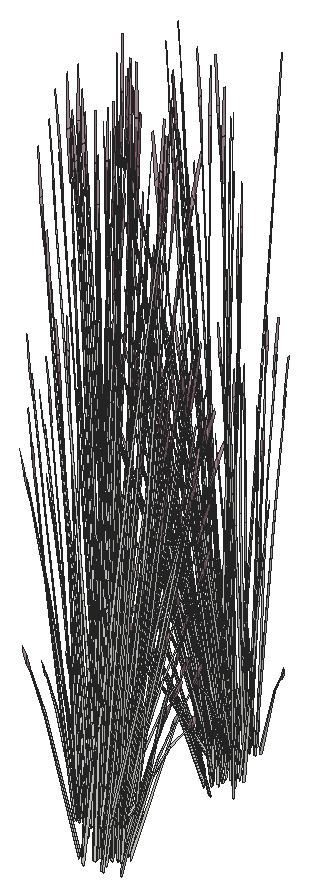
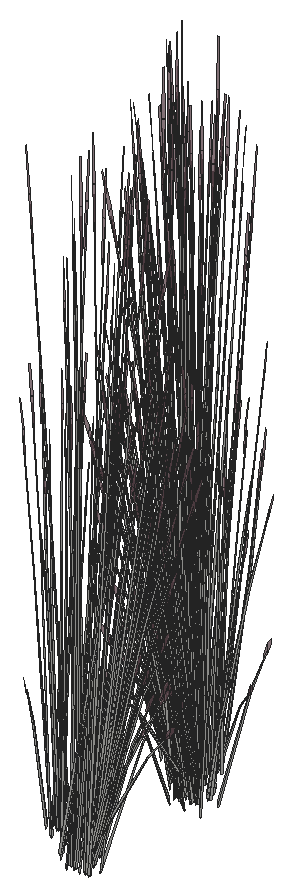
# SketchUp Ruby script. Lengths in inches.
U = 1.inch
M = Sketchup.active_model
def pt(a) = Geom::Point3d.new(a.map { |v| v * U })
def face(e, loops, mat)
  f = e.add_face(loops[0].map { |a| pt(a) })
  loops[1..].each { |l| e.add_face(l.map { |a| pt(a) }).erase! }
  f.material = f.back_material = mat if mat
  f
end
# faces: each face lists its corners as indices into pts; further lists are holes
def faces(e, pts, list, mat = nil) = list.each { |f| face(e, (f[0].is_a?(Array) ? f : [f]).map { |l| l.map { |i| pts[i] } }, mat) }
# xy, xz, yz: faces in a plane at the given z, y or x. An outline is a flat list of corners, or four numbers for a rectangle; further outlines are holes
def ring(l) = l.size == 4 ? [[l[0], l[1]], [l[2], l[1]], [l[2], l[3]], [l[0], l[3]]] : l.each_slice(2).to_a
def flat(e, list, mat, &to3) = list.each { |f| face(e, (f[0].is_a?(Array) ? f : [f]).map { |l| ring(l).map { |u, v| to3.(u, v) } }, mat) }
def xy(e, z, list, mat = nil) = flat(e, list, mat) { |x, y| [x, y, z] }
def xz(e, y, list, mat = nil) = flat(e, list, mat) { |x, z| [x, y, z] }
def yz(e, x, list, mat = nil) = flat(e, list, mat) { |y, z| [x, y, z] }
def lines(e, pts, list) = list.each { |a, b| e.add_line(pt(pts[a]), pt(pts[b])) }
# prism: a flat outline (further loops are holes) pulled along v
def prism(e, loops, v, mat = nil)
  f = face(e, loops, mat); d = Geom::Vector3d.new(v.map { |x| x * U })
  f.pushpull(f.normal.samedirection?(d) ? d.length : -d.length)
end
def box(e, o, s, mat = nil) = prism(e, [[o, [o[0] + s[0], o[1], o[2]], [o[0] + s[0], o[1] + s[1], o[2]], [o[0], o[1] + s[1], o[2]]]], [0, 0, s[2]], mat)
def at(x, y, z, deg = 0) = Geom::Transformation.translation(pt([x, y, z])) * Geom::Transformation.rotation(ORIGIN, Z_AXIS, deg.degrees)
def axes(o, x, y, z) = Geom::Transformation.new([*x, 0, *y, 0, *z, 0, *pt(o).to_a, 1])
def part(name) = M.definitions.add(name)
# library, detail: a bought-in or finely detailed component or shape, given as its bounding box
def library(name, o, s) = part(name).tap { |d| box(d.entities, o, s) }
def detail(e, o, s) = box(e.add_group.entities, o, s)
def put(e, d, t, mat = nil) = e.add_instance(d, t).tap { |i| i.material = mat if mat }
def group(e, t, mat = nil) = e.add_group.tap { |g| g.transformation = t; g.material = mat if mat }.entities
root = M.entities
M.materials.add("LightPink_Translucent").color = [144, 107, 117]
M.materials["LightPink_Translucent"].alpha = 0.75
c1 = part("blade")
p = [[2.15,0.21,22],[0,0.17,0],[0.09,0.45,0],[2.18,0.31,22],[2.29,0.31,22],[0.38,0.45,0],
  [2.48,0.24,33],[2.49,0.24,33],[2.48,0.22,33]]
faces(c1.entities,p,[[0,1,2,3],[4,5,2,3],[6,3,4,7],[8,0,3,6]])
c2 = part("seeds")
p = [[0.3,-0.1,1.38],[-0.01,-0.03,1.59],[-0.01,-0.03,0.03],[0.14,-0.07,-0.07],[0.29,-0.03,3],[0.15,0.01,3.11]]
faces(c2.entities,p,[[0,1,2,3],[1,0,4,5]],"LightPink_Translucent")
c3 = part("blade with seeds")
put(c3.entities,c1,at(0,0,0))
put(c3.entities,c2,axes([2.4,0.25,30.99],[1.5799,-0.05474,1.17369],[-0.12525,1.92788,0.29478],[-0.07173,-0.02425,1.56792]))
put(root,c3,axes([331.12,469.75,1400.36],[-0.29264,0.42323,0.45755],[-0.34767,-0.3736,0.17955],[0.07055,-0.04224,1.58856]))
put(root,c3,axes([331.44,470.5,1400.3],[-0.32829,-0.4014,-0.06131],[0.32849,-0.40164,0],[-0.01146,-0.01402,1.75571]))
put(root,c3,axes([330.61,469.05,1400.47],[-0.10196,0.46348,0.17642],[-0.3731,-0.13116,0.35086],[0.06445,-0.00226,1.60407]))
put(root,c3,axes([332.47,470.56,1403.05],[-0.29332,-0.1301,0.35414],[0.08555,-0.37955,-0.4572],[0.11809,-0.0348,0.87481]))
put(root,c3,axes([329.4,469.86,1402.73],[0.09971,-0.42522,0.48003],[0.32782,0.1454,0.3958],[-0.12892,0.02555,0.9933]))
put(root,c3,axes([330.46,469.42,1399.59],[-0.3474,0.18671,1.28929],[-0.11057,-0.53572,0.50096],[0.21332,0.00891,1.46642]))
put(root,c3,axes([331.39,469.56,1400.62],[0.06809,-0.4162,0.1448],[0.33266,0.07225,-0.41347],[0.06054,0.04274,1.26744]))
put(root,c3,axes([329.37,469.75,1402.73],[-0.12963,-0.31798,0.0643],[0.23638,-0.15564,0.50621],[-0.1042,0.03071,0.77189]))
put(root,c3,axes([330.82,470.55,1400.36],[0.44609,0.09826,0.45755],[-0.09078,0.55493,0.17955],[-0.06519,-0.05359,1.58856]))
put(root,c3,axes([333.17,470.15,1399.49],[-0.01845,-0.0708,1.76342],[0.12793,-0.41416,-0.26939],[0.12905,-0.00596,0.30037]))
put(root,c3,axes([329.36,470.08,1399.49],[0.00895,0.0735,1.76342],[-0.18044,0.38382,-0.26939],[-0.12817,-0.01935,0.30037]))
put(root,c3,axes([331.25,469.67,1400.72],[-0.21202,-0.39143,0.44739],[0.32115,-0.27564,-0.21531],[0.06861,0.04843,1.43643]))
put(root,c3,axes([330.15,471.46,1400.03],[-0.08291,-0.40636,-0.30978],[0.32928,-0.11539,0.30978],[-0.06638,-0.04686,1.38974]))
put(root,c3,axes([330.58,471.44,1400.47],[0.37926,-0.12378,0.17642],[0.09365,0.46065,0.35086],[-0.03382,-0.06712,1.60407]))
put(root,c3,axes([331.36,469.7,1400.67],[0.35635,-0.30962,-0.29095],[0.23697,0.43749,-0.50002],[0.08792,0.04443,1.59708]))
put(root,c3,axes([332.78,470.52,1402.53],[0.29332,0.1301,-0.35414],[-0.08555,0.37955,0.4572],[0.11809,-0.0348,0.87481]))
put(root,c3,axes([330.0625,471.64,1400.02],[-0.33032,-0.23318,-0.49651],[0.19744,-0.41812,0],[-0.07523,-0.05311,1.57504]))
put(root,c3,axes([332.26,468.88,1400.02],[0.33032,0.23318,-0.49651],[-0.19744,0.41812,0],[0.07523,0.05311,1.57504]))
put(root,c3,axes([329.33,469.91,1402.53],[-0.29332,-0.1301,-0.35414],[0.08555,-0.37955,0.4572],[-0.11809,0.0348,0.87481]))
put(root,c3,axes([331.63,470.21,1400.21],[0.39487,0,0],[0,0.48281,0],[0,0,1.78407]))
put(root,c3,axes([330.96,470.82,1400.67],[-0.35635,0.30962,-0.29095],[-0.23697,-0.43749,-0.50002],[-0.08792,-0.04443,1.59708]))
put(root,c3,axes([331.74,469.08,1400.47],[-0.37926,0.12378,0.17642],[-0.09365,-0.46065,0.35086],[0.03382,0.06712,1.60407]))
put(root,c3,axes([331.98,470.05,1401.875],[-0.14639,0.01056,1.71376],[0.09712,-0.45778,0.13857],[0.20862,0.02831,0.73262]))
put(root,c3,axes([332.17,469.05,1400.03],[0.08291,0.40636,-0.30978],[-0.32928,0.11539,0.30978],[0.06638,0.04686,1.38974]))
put(root,c3,axes([332.73,470.68,1402.73],[0.12963,0.31798,0.0643],[-0.23638,0.15564,0.50621],[0.1042,-0.03071,0.77189]))
put(root,c3,axes([331.5,469.96,1400.38],[-0.44609,-0.09826,0.49198],[0.09078,-0.55493,0.19306],[0.06519,0.05359,1.70813]))
put(root,c3,axes([332.71,470.5625,1402.73],[-0.09971,0.42522,0.48003],[-0.32782,-0.1454,0.3958],[0.12892,-0.02555,0.9933]))
put(root,c3,axes([331.15,471.33,1400.2],[-0.11516,-0.40207,0],[0.32884,-0.1408,0],[0,0,1.54371]))
put(root,c3,axes([330.93,470.95,1400.62],[-0.06809,0.4162,0.1448],[-0.33266,-0.07225,-0.41347],[-0.06054,-0.04274,1.26744]))
put(root,c3,axes([329.64,469.87,1403.05],[0.29332,0.1301,0.35414],[-0.08555,0.37955,-0.4572],[-0.11809,0.0348,0.87481]))
put(root,c3,axes([331.58,471.27,1400.18],[0.37054,-0.15823,-0.19198],[0.1302,0.45581,0.00008],[0.0409,-0.01749,1.73897]))
put(root,c3,axes([331.71,471.47,1400.47],[0.10196,-0.46348,0.17642],[0.3731,0.13116,0.35086],[-0.06445,0.00226,1.60407]))
put(root,c3,axes([331.62,470.41,1400.21],[0.24637,0.30123,0],[-0.24637,0.30123,0],[0,0,1.69266]))
put(root,c3,axes([330.22,469.85,1401.34],[0.10032,-0.06746,1.77064],[0.0346,0.47103,0.13857],[-0.2173,0.0625,0.63284]))
put(root,c3,axes([332.29,470.28,1400.47],[-0.2773,-0.3397,0.17642],[0.27945,-0.32949,0.35086],[-0.03063,0.06937,1.60407]))
put(root,c3,axes([331.78,469.77,1400.06],[0.36714,0.07646,-0.62353],[-0.07747,0.47163,-0.16365],[0.10956,0.05715,1.37633]))
put(root,c3,axes([333.4,470.59,1400.77],[-0.21807,0.07699,1.1486],[0.10265,-0.31819,0.84392],[0.11568,0.02177,0.25299]))
put(root,c3,axes([331.07,471.51,1400.2],[-0.35581,-0.20937,0],[0.17124,-0.43505,0],[0,0,1.62707]))
put(root,c3,axes([331.36,470.96,1400.46],[-0.34464,-0.37536,-0.25192],[0.29,-0.42149,0.5513],[-0.0928,0.04391,1.68216]))
put(root,c3,axes([330.45,471.68,1400.48],[0.33032,0.23318,0.49651],[-0.19744,0.41812,0],[-0.07523,-0.05311,1.57504]))
put(root,c3,axes([331.62,470.0625,1400.72],[0.17124,-0.42022,0.44739],[0.35581,0.20224,-0.21531],[0,0.09687,1.43643]))
put(root,c3,axes([333.3,471.94,1402.71],[-0.03191,-0.04083,1.77383],[0.06981,-0.43764,-0.16761],[0.12571,-0.02796,0.31391]))
put(root,c3,axes([329.14,470.16,1402.72],[-0.05763,0.06055,1.74944],[0.0049,0.44239,-0.27667],[-0.13211,0.05753,0.14031]))
put(root,c3,axes([331.55,470.3,1400.29],[0,0.53934,-0.05637],[-0.44133,0,0],[0,0.01695,1.79368]))
put(root,c3,axes([329.53,470.11,1402.68],[-0.09562,0.42421,-0.51099],[-0.32782,-0.1454,-0.3958],[-0.13199,0.0389,0.97773]))
put(root,c3,axes([329.51,469.74,1403.03],[0.17758,0.42229,-0.1216],[-0.31518,0.20752,-0.67495],[-0.13282,0.05572,1.02557]))
put(root,c3,axes([331.58,469.92,1400.21],[0.21202,0.39143,-0.44739],[-0.32115,0.27564,0.21531],[0.06861,0.04843,1.43643]))
put(root,c3,axes([333.02,471.57,1401.93],[-0.06755,-0.39203,-0.03492],[0.31928,-0.09013,-0.15832],[0.06667,0.02485,0.52218]))
put(root,c3,axes([330.26,471.92,1400.375],[-0.22066,0.46731,0],[-0.36918,-0.26061,-0.51607],[-0.08408,-0.05936,1.63711]))
put(root,c3,axes([332.19,471.5625,1403.03],[0.0189,-0.47427,-0.1216],[0.35781,0.01296,-0.67495],[0.13781,0.03295,1.02557]))
put(root,c3,axes([332.52,470.3,1400.48],[0,-0.46636,0.49651],[0.39487,0,0],[0,0.10622,1.57504]))
put(root,c3,axes([331.53,470.64,1400.72],[0.38326,-0.02879,0.44739],[0.03466,0.47788,-0.21531],[-0.06861,0.04843,1.43643]))
put(root,c3,axes([331.77,470.16,1400.62],[0.32884,-0.136,0.1448],[0.11516,0.38837,-0.41347],[0,0.08547,1.26744]))
put(root,c3,axes([332.14,471.38,1403.05],[-0.20082,-0.29199,0.35414],[0.2293,-0.2764,-0.4572],[0.1165,0.04206,0.87481]))
put(root,c3,axes([331.1875,470.875,1400.21],[-0.38326,0.02879,-0.44739],[-0.03466,-0.47788,0.21531],[-0.06861,0.04843,1.43643]))
put(root,c3,axes([332.99,471.1,1400.59],[-0.085,-0.1147,1.43002],[0.1106,-0.37943,-0.30754],[0.17198,0.0514,0.61141]))
put(root,c3,axes([331.47,471.52,1400.2],[0.35581,0.20937,0],[-0.17124,0.43505,0],[0,0,1.74954]))
put(root,c3,axes([332.5,471.28,1402.72],[0.07571,-0.00789,1.74944],[0.20767,-0.36231,-0.27667],[0.13467,0.04783,0.14031]))
put(root,c3,axes([331.61,471.98,1400.19],[-0.21791,-0.46895,-0.05142],[0.36918,-0.26061,0.51607],[-0.09097,0.04465,1.6363]))
put(root,c3,axes([331.53,470.85,1400.62],[0.26075,0.2802,0.1448],[-0.2175,0.31612,-0.41347],[-0.06054,0.04274,1.26744]))
put(root,c3,axes([329.47,470.92,1402.73],[-0.08753,-0.42921,0.48003],[0.34336,-0.07449,0.3958],[-0.1012,0.10094,0.9933]))
put(root,c3,axes([329.41,470.84,1402.73],[-0.2423,-0.19613,0.0643],[0.14107,-0.2793,0.50621],[-0.07768,0.0903,0.77189]))
put(root,c3,axes([329.52,470.32,1401.875],[0.12246,-0.09864,1.71376],[0.1031,0.45582,0.13857],[-0.19225,0.10302,0.73262]))
put(root,c3,axes([332.21,471.33,1402.98],[0.35281,0.01123,-0.71045],[-0.0237,0.47284,0.08574],[0.14947,0.0499,1.00501]))
put(root,c3,axes([331.8125,471.71,1400.48],[0.33032,-0.23318,0.49651],[0.19744,0.41812,0],[-0.07523,0.05311,1.57504]))
put(root,c3,axes([331.34,471.35,1400.29],[0.15345,0.53576,-0.06012],[-0.43845,0.18773,0],[0.00536,0.01871,1.72173]))
put(root,c3,axes([331.51,471.93,1400.03],[-0.32928,-0.11539,-0.30978],[0.08291,-0.40636,0.30978],[-0.06638,0.04686,1.38974]))
put(root,c3,axes([329.14,471.1,1400.59],[0.12266,0.03828,1.43002],[0.07906,0.39104,-0.30754],[-0.16661,0.0732,0.61141]))
put(root,c3,axes([329.6875,470.78,1403.05],[0.30722,-0.06665,0.35414],[0.08112,0.381,-0.4572],[-0.08804,0.10234,0.87481]))
put(root,c3,axes([332.78,470.375,1400.375],[0.44133,0,0],[0,0.52122,-0.51607],[0,0.11871,1.63711]))
put(root,c3,axes([328.5,470.61,1402.71],[0.04504,0.01251,1.77383],[0.13934,0.41205,-0.16761],[-0.0922,0.10815,0.31391]))
put(root,c3,axes([332.61,470.64,1400.2],[-0.44111,-0.00373,-0.04976],[0,-0.52122,0.49943],[-0.01386,0.11865,1.58352]))
put(root,c3,axes([331.65,470.1875,1400.67],[0.39748,0.22252,-0.29095],[-0.19139,0.46966,-0.50002],[0.01249,0.11531,1.59708]))
put(root,c3,axes([328.88,471.92,1400.77],[0.14709,-0.21136,1.1486],[0.05804,0.3346,0.84392],[-0.1063,0.05991,0.25299]))
put(root,c3,axes([332.42,471.53,1402.53],[0.20082,0.29199,-0.35414],[-0.2293,0.2764,0.4572],[0.1165,0.04206,0.87481]))
put(root,c3,axes([332.52,470.72,1400.03],[-0.24637,0.29097,-0.30978],[-0.24637,-0.29097,0.30978],[0,0.09372,1.38974]))
put(root,c3,axes([331.46,470.75,1400.67],[0.04113,0.53214,-0.29095],[-0.42835,0.03218,-0.50002],[-0.07543,0.07088,1.59708]))
put(root,c3,axes([332.32,471.64,1402.73],[-0.01777,0.35463,0.0643],[-0.26836,-0.00972,0.50621],[0.1028,0.03711,0.77189]))
put(root,c3,axes([331.61,470.54,1400.21],[-0.17124,0.42022,-0.44739],[-0.35581,-0.20224,0.21531],[0,0.09687,1.43643]))
put(root,c3,axes([329.43,471.01,1402.53],[-0.30722,0.06665,-0.35414],[-0.08112,-0.381,0.4572],[-0.08804,0.10234,0.87481]))
put(root,c3,axes([332.34,471.53,1402.73],[-0.26024,0.30729,0.48003],[-0.22444,-0.32634,0.3958],[0.1221,0.05668,0.9933]))
put(root,c3,axes([328.99,471.86,1403.65],[0.31145,0.12449,-0.06488],[-0.0958,0.38314,-0.29416],[-0.05094,0.05817,0.97024]))
put(root,c3,axes([331.2,471.15,1400.06],[-0.23773,0.35053,-0.62353],[-0.29532,-0.31785,-0.16365],[-0.09526,0.08744,1.37633]))
put(root,c3,axes([331.52,471.88,1403.05],[-0.05451,-0.37564,0.35414],[0.31161,-0.09919,-0.4572],[0.0837,0.10765,0.87481]))
put(root,c3,axes([331.62,471.74,1400.33],[0.44186,0.15158,0.30756],[-0.11054,0.54181,-0.36492],[-0.07313,0.06781,1.64885]))
put(root,c3,axes([331.59,472.11,1400.02],[-0.33032,0.23318,-0.49651],[-0.19744,-0.41812,0],[-0.07523,0.05311,1.57504]))
put(root,c3,axes([332.6875,470.73,1400.02],[0,0.46636,-0.49651],[-0.39487,0,0],[0,0.10622,1.57504]))
put(root,c3,axes([331.7,470.78,1401.875],[-0.1311,-0.08035,1.71376],[0.27131,-0.33708,0.13857],[0.16909,0.15206,0.73262]))
put(root,c3,axes([331.72,469.72,1402.47],[-0.30498,-0.24231,1.38283],[0.32203,-0.37727,0.59665],[0.0984,0.22736,1.33663]))
put(root,c3,axes([329.53,470.75,1403.03],[0.32648,0.25715,-0.1216],[-0.18809,0.3724,-0.67495],[-0.09224,0.12945,1.02557]))
put(root,c3,axes([332.18,471.7,1400.77],[-0.19872,-0.13409,1.1486],[0.2566,-0.13625,0.84392],[0.06921,0.11541,0.25299]))
put(root,c3,axes([331.49,472.08,1403.03],[0.21031,-0.39918,-0.1216],[0.30457,0.22997,-0.67495],[0.10587,0.11278,1.02557]))
put(root,c3,axes([329.97,470.63,1401.875],[0.08815,-0.14329,1.71376],[0.22258,0.38678,0.13857],[-0.15267,0.17614,0.73262]))
put(root,c3,axes([329.6875,471.05,1402.68],[0.09067,0.42583,-0.51099],[-0.34336,0.07449,-0.3958],[-0.0984,0.11438,0.97773]))
put(root,c3,axes([330.1,471.54,1403.05],[0.23881,-0.24554,0.35414],[0.22606,0.28036,-0.4572],[-0.0344,0.14245,0.87481]))
put(root,c3,axes([331.89,472.04,1400.375],[0.22066,0.46731,0],[-0.36918,0.26061,-0.51607],[-0.08408,0.05936,1.63711]))
put(root,c3,axes([331.21,472.41,1402.71],[0.00104,-0.05646,1.77383],[0.30246,-0.2491,-0.16761],[0.10506,0.08891,0.31391]))
put(root,c3,axes([332.24,472.19,1399.49],[0.02571,-0.06733,1.76342],[0.32373,-0.19829,-0.26939],[0.09815,0.10263,0.30037]))
put(root,c3,axes([331.7,470.1875,1400.84],[-0.00964,-0.43909,1.41272],[0.43635,0.11382,0.59816],[-0.1032,0.24027,1.3335]))
put(root,c3,axes([331.8125,470.67,1400.09],[0.12941,0.42699,-0.69212],[-0.37279,0.15378,-0.18165],[0.0143,0.14459,1.52773]))
put(root,c3,axes([329.88,471.76,1402.73],[-0.29004,-0.02173,0.0643],[0.00795,-0.32812,0.50621],[-0.03035,0.12569,0.77189]))
put(root,c3,axes([329.27,472.14,1399.49],[0.04734,0.04659,1.76342],[0.08027,0.4317,-0.26939],[-0.10492,0.09206,0.30037]))
put(root,c3,axes([329.98,471.79,1402.73],[-0.25132,-0.3182,0.48003],[0.2669,-0.27442,0.3958],[-0.04636,0.14929,0.9933]))
put(root,c3,axes([331.74,471.88,1402.68],[0.34827,-0.11086,-0.51099],[0.06092,0.41983,-0.3958],[0.09354,0.12031,0.97773]))
put(root,c3,axes([330.77,471.94,1403.05],[0.1064,-0.35863,0.35414],[0.31043,0.1046,-0.4572],[0.02846,0.14439,0.87481]))
put(root,c3,axes([332.22,472.31,1400.67],[-0.22633,-0.01463,1.0506],[0.14947,-0.31064,0.58006],[0.08941,0.11036,0.8241]))
put(root,c3,axes([331.56,472.22,1402.73],[-0.16041,0.29625,0.0643],[-0.22843,-0.17248,0.50621],[0.07385,0.09498,0.77189]))
put(root,c3,axes([331.1875,473.22,1403.65],[0.2439,-0.26754,-0.06488],[0.22348,0.29302,-0.29416],[0.01573,0.08303,0.97024]))
put(root,c3,axes([331.63,472.14,1402.73],[-0.35104,0.10702,0.48003],[-0.06092,-0.41983,0.3958],[0.08256,0.12373,0.9933]))
put(root,c3,axes([329.9,470.98,1401.875],[0.06572,-0.16029,1.71376],[0.27569,0.33172,0.13857],[-0.12437,0.20675,0.73262]))
put(root,c3,axes([331.48,471.55,1400.59],[0.00623,-0.15459,1.43002],[0.29764,-0.17268,-0.30754],[0.09188,0.18503,0.61141]))
put(root,c3,axes([330.67,472.27,1402.73],[-0.26007,0.1585,0.0643],[-0.12729,-0.28902,0.50621],[0.02512,0.1274,0.77189]))
put(root,c3,axes([329.98,471.89,1402.53],[-0.23881,0.24554,-0.35414],[-0.22606,-0.28036,0.4572],[-0.0344,0.14245,0.87481]))
put(root,c3,axes([329.15,471.82,1402.72],[-0.00877,0.09229,1.74944],[0.24897,0.32105,-0.27667],[-0.06518,0.15182,0.14031]))
put(root,c3,axes([329.95,471.61,1403.4],[0.3879,0.02311,-0.13498],[-0.0106,0.43749,-0.74919],[-0.02694,0.1685,1.13838]))
put(root,c3,axes([330.67,472.1,1403.03],[0.34538,-0.21713,-0.1216],[0.16972,0.38536,-0.67495],[0.04557,0.16239,1.02557]))
put(root,c3,axes([330.77,472.24,1403.0625],[-0.34777,-0.12192,0.53283],[0.11892,-0.40083,0.43934],[0.0209,0.15763,1.10256]))
put(root,c3,axes([330.13,472.84,1400.77],[-0.00913,-0.2773,1.1486],[0.22824,0.19778,0.84392],[-0.04489,0.13217,0.25299]))
put(root,c3,axes([330.73,472.18,1399.49],[0.05712,-0.02538,1.76342],[0.34359,0.13968,-0.26939],[0.01005,0.15742,0.30037]))
put(root,c3,axes([330.21,471.77,1403],[0.25266,0.31335,-0.5672],[-0.2669,0.27442,-0.43934],[-0.03844,0.15921,1.08528]))
put(root,c3,axes([329.9375,472.24,1400.82],[0.32063,-0.08258,0.06507],[0.07371,0.33271,-0.86304],[-0.02033,0.16842,0.7736]))
put(root,c3,axes([330.96,472.08,1402.68],[0.34695,0.11691,-0.51099],[-0.11892,0.40083,-0.3958],[0.03181,0.16138,0.97773]))
put(root,c3,axes([331.16,471.25,1401.875],[-0.08068,-0.14973,1.71376],[0.3728,-0.12606,0.13857],[0.08426,0.23506,0.73262]))
put(root,c3,axes([330.8,472.32,1402.53],[-0.1064,0.35863,-0.35414],[-0.31043,-0.1046,0.4572],[0.02846,0.14439,0.87481]))
put(root,c3,axes([330.13,471.63,1403.34],[-0.00918,0.43138,-0.7886],[-0.38672,-0.02897,0.09517],[-0.04081,0.18275,1.11556]))
put(root,c3,axes([329.125,472.76,1402.71],[0.04004,-0.02816,1.77383],[0.33095,0.18728,-0.16761],[-0.00778,0.15594,0.31391]))
put(root,c3,axes([330.5,471.32,1401.875],[-0.00864,-0.17899,1.71376],[0.37441,0.11874,0.13857],[-0.02316,0.25508,0.73262]))
put(root,c3,axes([330.84,472,1402.98],[0.16845,0.3792,-0.71045],[-0.34676,0.21133,0.08574],[0.03939,0.18322,1.00501]))
put(root,c3,axes([329.86,472.6,1400.59],[0.11138,-0.07357,1.43002],[0.27499,0.22183,-0.30754],[-0.08185,0.19194,0.61141]))
put(root,c3,axes([330.58,472.96,1402.72],[0.04474,0.0751,1.74944],[0.36104,0.0295,-0.27667],[0.03631,0.16562,0.14031]))
put(root,c3,axes([330.01,472.24,1401.36],[0.00775,-0.24075,1.54345],[0.34877,0.12716,0.21329],[-0.03022,0.25658,0.72882]))
put(root,c3,axes([330.27,483.48,1401.875],[0.08068,0.14973,1.71376],[-0.3728,0.12606,0.13857],[-0.08426,-0.23506,0.73262]))
put(root,c3,axes([330.89,482.49,1402.72],[-0.05398,-0.06539,1.74944],[-0.36026,0.04145,-0.27667],[-0.0575,-0.15639,0.14031]))
put(root,c3,axes([331.72,483.27,1400.59],[-0.10032,0.0944,1.43002],[-0.30046,-0.16522,-0.30754],[0.05569,-0.20547,0.61141]))
put(root,c3,axes([331.27,483.59,1402.98],[-0.16845,-0.3792,-0.71045],[0.34676,-0.21133,0.08574],[-0.03939,-0.18322,1.00501]))
put(root,c3,axes([330.17,483.09,1400.59],[-0.02137,0.15256,1.43002],[-0.31245,0.12771,-0.30754],[-0.07303,-0.19719,0.61141]))
put(root,c3,axes([330.98,482.75,1399.49],[-0.0592,0.0168,1.76342],[-0.32738,-0.18913,-0.26939],[0.00549,-0.15776,0.30037]))
put(root,c3,axes([331.97,483.97,1402.98],[0.00918,-0.43138,-0.71045],[0.38672,0.02897,0.08574],[0.04081,-0.18275,1.00501]))
put(root,c3,axes([332.51,483.29,1402.72],[-0.00341,-0.09282,1.74944],[-0.28775,-0.26825,-0.27667],[0.04449,-0.16261,0.14031]))
put(root,c3,axes([331.3,483.27,1402.53],[0.1064,-0.35863,-0.35414],[0.31043,0.1046,0.4572],[-0.02846,-0.14439,0.87481]))
put(root,c3,axes([331.53,483.75,1401.875],[-0.06572,0.16029,1.71376],[-0.27569,-0.33172,0.13857],[0.12437,-0.20675,0.73262]))
put(root,c3,axes([332.43,482.96,1402.71],[-0.03584,0.03562,1.77383],[-0.35118,-0.12018,-0.16761],[-0.01271,-0.15545,0.31391]))
put(root,c3,axes([331.14,483.52,1402.68],[-0.34695,-0.11691,-0.51099],[0.11892,-0.40083,-0.3958],[-0.03181,-0.16138,0.97773]))
put(root,c3,axes([331.35,482.51,1400.77],[0.04528,0.27194,1.1486],[-0.25117,-0.15062,0.84392],[0.02703,-0.13924,0.25299]))
put(root,c3,axes([331.89,483.82,1402.68],[-0.25266,-0.31335,-0.51099],[0.2669,-0.27442,-0.3958],[0.03844,-0.15921,0.97773]))
put(root,c3,axes([330.52,482.28,1402.71],[-0.00658,0.0559,1.77383],[-0.32474,0.20287,-0.16761],[-0.09556,-0.1037,0.31391]))
put(root,c3,axes([330.45,483.27,1403.09],[0.39316,-0.11987,0.53763],[0.06823,0.47021,0.4433],[-0.09247,-0.13858,1.11249]))
put(root,c3,axes([331.34,483.36,1402.73],[0.34777,0.12192,0.48003],[-0.11892,0.40083,0.3958],[-0.0209,-0.15763,0.9933]))
put(root,c3,axes([331.4375,483.5,1403.03],[-0.34538,0.21713,-0.1216],[-0.16972,-0.38536,-0.67495],[-0.04557,-0.16239,1.02557]))
put(root,c3,axes([332.15,483.99,1403.03],[-0.3879,-0.02311,-0.1216],[0.0106,-0.43749,-0.67495],[0.02694,-0.1685,1.02557]))
put(root,c3,axes([332.13,483.71,1402.53],[0.23881,-0.24554,-0.35414],[0.22606,0.28036,0.4572],[0.0344,-0.14245,0.87481]))
put(root,c3,axes([330.0625,482.84,1400.77],[0.18411,0.16231,1.1486],[-0.26813,0.09757,0.84392],[-0.05737,-0.12474,0.25299]))
put(root,c3,axes([331.43,483.33,1402.73],[0.26007,-0.1585,0.0643],[0.12729,0.28902,0.50621],[-0.02512,-0.1274,0.77189]))
put(root,c3,axes([330.51,483.7,1402.98],[-0.30095,-0.22541,-0.71045],[0.21388,-0.395,0.08574],[-0.10904,-0.13459,1.00501]))
put(root,c3,axes([330.4,483.4,1402.53],[-0.05451,-0.37564,-0.35414],[0.31161,-0.09919,0.4572],[-0.0837,-0.10765,0.87481]))
put(root,c3,axes([330.54,483.37,1402.73],[0.16041,-0.29625,0.0643],[0.22843,0.17248,0.50621],[-0.07385,-0.09498,0.77189]))
put(root,c3,axes([329.92,483.33,1399.49],[-0.03419,0.06144,1.76342],[-0.3455,0.13246,-0.26939],[-0.08346,-0.12049,0.30037]))
put(root,c3,axes([330.49,485.02,1400.1],[-0.14494,-0.47823,-0.69835],[0.41752,-0.17223,-0.18329],[-0.01602,-0.16194,1.54149]))
put(root,c3,axes([329.73,483.95,1401.875],[0.1311,0.08035,1.71376],[-0.27131,0.33708,0.13857],[-0.16909,-0.15206,0.73262]))
put(root,c3,axes([332.43,483.56,1399.49],[-0.05283,-0.03674,1.76342],[-0.13569,-0.41045,-0.26939],[0.09154,-0.11138,0.30037]))
put(root,c3,axes([331.33,483.65,1403.05],[-0.1064,0.35863,0.35414],[-0.31043,-0.1046,-0.4572],[-0.02846,-0.14439,0.87481]))
put(root,c3,axes([330.37,483.71,1402.68],[-0.34827,0.11086,-0.51099],[-0.06092,-0.41983,-0.3958],[-0.09354,-0.12031,0.97773]))
put(root,c3,axes([332.125,483.8,1402.73],[0.25132,0.3182,0.48003],[-0.2669,0.27442,0.3958],[0.04636,-0.14929,0.9933]))
put(root,c3,axes([330.61,483.34,1403.43],[-0.23555,0.44708,-0.13619],[-0.34112,-0.25757,-0.75594],[-0.11858,-0.12631,1.14864]))
put(root,c3,axes([332.22,483.83,1402.73],[0.29004,0.02173,0.0643],[-0.00795,0.32812,0.50621],[0.03035,-0.12569,0.77189]))
put(root,c3,axes([332,484.05,1403.05],[-0.23881,0.24554,0.35414],[-0.22606,-0.28036,-0.4572],[0.0344,-0.14245,0.87481]))
put(root,c3,axes([332.42,484.72,1402.98],[0.18436,-0.36797,-0.71045],[0.32306,0.26151,0.08574],[0.11008,-0.13332,1.00501]))
put(root,c3,axes([330.43,483.64,1400.375],[-0.22066,-0.46731,0],[0.36918,-0.26061,-0.51607],[0.08408,-0.05936,1.63711]))
put(root,c3,axes([332.41,484.54,1402.68],[-0.09067,-0.42583,-0.51099],[0.34336,-0.07449,-0.3958],[0.0984,-0.11438,0.97773]))
put(root,c3,axes([330.92,483.08,1400.13],[-0.2439,0.26754,-0.03893],[-0.22348,-0.29302,-0.17649],[-0.01573,-0.08303,0.58215]))
put(root,c3,axes([329.71,483.21,1402.72],[-0.07594,-0.00329,1.74944],[-0.24177,0.32918,-0.27667],[-0.129,-0.06726,0.14031]))
put(root,c3,axes([332.58,484.85,1403.03],[-0.32648,-0.25715,-0.1216],[0.18809,-0.3724,-0.67495],[0.09224,-0.12945,1.02557]))
put(root,c3,axes([331.23,486.25,1401.33],[0.305,0.18805,1.51261],[-0.29879,0.40513,0.59816],[-0.13384,-0.24012,1.26806]))
put(root,c3,axes([330.59,483.71,1403.05],[0.05451,0.37564,0.35414],[-0.31161,0.09919,-0.4572],[-0.0837,-0.10765,0.87481]))
put(root,c3,axes([329.63,484.95,1400.02],[0,-0.46636,-0.49651],[0.39487,0,0],[0,-0.10622,1.57504]))
put(root,c3,axes([330.73,483.57,1400.02],[0.33032,-0.23318,-0.49651],[0.19744,0.41812,0],[0.07523,-0.05311,1.57504]))
put(root,c3,axes([332.69,484.38,1400.59],[-0.12609,-0.01381,1.43002],[-0.12917,-0.37055,-0.30754],[0.1549,-0.10482,0.61141]))
put(root,c3,axes([329.65,483.95,1403.09],[0.29147,-0.34417,0.53763],[0.25138,0.3655,0.4433],[-0.13675,-0.06349,1.11249]))
put(root,c3,axes([333.38,484.74,1402.71],[-0.0461,-0.00354,1.77383],[-0.19143,-0.37951,-0.16761],[0.07688,-0.12478,0.31391]))
put(root,c3,axes([331.12,484.53,1400.06],[0.23773,-0.35053,-0.62353],[0.29532,0.31785,-0.16365],[0.09526,-0.08744,1.37633]))
put(root,c3,axes([332.84,483.7,1400.77],[-0.11756,0.2374,1.1486],[-0.10105,-0.31895,0.84392],[0.09709,-0.07992,0.25299]))
put(root,c3,axes([332.67,484.59,1402.53],[0.30722,-0.06665,-0.35414],[0.08112,0.381,0.4572],[0.08804,-0.10234,0.87481]))
put(root,c3,axes([329.78,483.95,1402.73],[0.01777,-0.35463,0.0643],[0.26836,0.00972,0.50621],[-0.1028,-0.03711,0.77189]))
put(root,c3,axes([330.71,485.14,1400.21],[0.17124,-0.42022,-0.44739],[0.35581,0.20224,0.21531],[0,-0.09687,1.43643]))
put(root,c3,axes([329.68,484.06,1402.53],[-0.20082,-0.29199,-0.35414],[0.2293,-0.2764,0.4572],[-0.1165,-0.04206,0.87481]))
put(root,c3,axes([330.86,484.93,1400.67],[-0.04113,-0.53214,-0.29095],[0.42835,-0.03218,-0.50002],[0.07543,-0.07088,1.59708]))
put(root,c3,axes([329.8,484.96,1400.03],[0.24637,-0.29097,-0.30978],[0.24637,0.29097,0.30978],[0,-0.09372,1.38974]))
put(root,c3,axes([329.7,483.57,1400.13],[-0.10181,0.3808,-0.03893],[-0.31336,-0.11714,-0.17649],[-0.04758,-0.06228,0.58215]))
put(root,c3,axes([332.42,484.8125,1403.05],[-0.30722,0.06665,0.35414],[-0.08112,-0.381,-0.4572],[0.08804,-0.10234,0.87481]))
put(root,c3,axes([330.67,485.49,1400.67],[-0.39748,-0.22252,-0.29095],[0.19139,-0.46966,-0.50002],[-0.01249,-0.11531,1.59708]))
put(root,c3,axes([329.53,485.31,1400.375],[-0.44133,0,0],[0,-0.52122,-0.51607],[0,-0.11871,1.63711]))
put(root,c3,axes([329.61,484.375,1400.59],[0.06891,0.12984,1.43002],[-0.15879,0.35293,-0.30754],[-0.16304,-0.08436,0.61141]))
put(root,c3,axes([330.81,483.76,1400.03],[0.32928,0.11539,-0.30978],[-0.08291,0.40636,0.30978],[0.06638,-0.04686,1.38974]))
put(root,c3,axes([329.89,484.26,1402.98],[-0.35281,-0.01123,-0.71045],[0.0237,-0.47284,0.08574],[-0.14947,-0.0499,1.00501]))
put(root,c3,axes([332.7,484.75,1402.73],[0.2423,0.19613,0.0643],[-0.14107,0.2793,0.50621],[0.07768,-0.0903,0.77189]))
put(root,c3,axes([332.63,484.67,1402.73],[0.08753,0.42921,0.48003],[-0.34336,0.07449,0.3958],[0.1012,-0.10094,0.9933]))
put(root,c3,axes([333.55,485.19,1402.72],[0.04898,-0.07104,1.74944],[-0.06269,-0.43574,-0.27667],[0.12289,-0.08262,0.14031]))
put(root,c3,axes([329.875,485.17,1400.33],[-0.32829,0.39208,0.30756],[-0.32849,-0.38796,-0.36492],[-0.01146,-0.11134,1.64885]))
put(root,c3,axes([329.42,483.49,1402.71],[0.02617,0.04654,1.77383],[-0.12614,0.41836,-0.16761],[-0.12775,0.00303,0.31391]))
put(root,c3,axes([330.92,485.35,1400.43],[0.39767,0.22603,0.24065],[-0.19139,0.46966,0.50002],[0,-0.10827,1.60543]))
put(root,c3,axes([330.77,485.99,1400.4375],[0.09355,-0.55261,-0.23429],[0.44354,0.09633,0.51271],[-0.0775,-0.07631,1.5644]))
put(root,c3,axes([329.78,484.36,1402.68],[-0.25628,0.30892,-0.51099],[-0.22444,-0.32634,-0.3958],[-0.13021,-0.047,0.97773]))
put(root,c3,axes([329.97,484.22,1403.05],[0.20082,0.29199,0.35414],[-0.2293,0.2764,-0.4572],[-0.1165,-0.04206,0.87481]))
put(root,c3,axes([329.2,484.76,1400.77],[0.22533,-0.03337,1.1486],[-0.14293,0.29403,0.84392],[-0.11135,-0.04411,0.25299]))
put(root,c3,axes([330.79,485.04,1400.72],[-0.38326,0.02879,0.44739],[-0.03466,-0.47788,-0.21531],[0.06861,-0.04843,1.43643]))
put(root,c3,axes([329.91,484.03,1403.03],[-0.0189,0.47427,-0.1216],[-0.35781,-0.01296,-0.67495],[-0.13781,-0.03295,1.02557]))
put(root,c3,axes([329.8,485.39,1400.48],[0,0.46636,0.49651],[-0.39487,0,0],[0,-0.10622,1.57504]))
put(root,c3,axes([332.59,485.85,1403.03],[-0.17758,-0.42229,-0.1216],[0.31518,-0.20752,-0.67495],[0.13282,-0.05572,1.02557]))
put(root,c3,axes([332.57,485.49,1402.68],[0.09562,-0.42421,-0.51099],[0.32782,0.1454,-0.3958],[0.13199,-0.0389,0.97773]))
put(root,c3,axes([332.06,483.76,1400.375],[0.22066,-0.46731,0],[0.36918,0.26061,-0.51607],[0.08408,0.05936,1.63711]))
put(root,c3,axes([329.46,484.69,1401.875],[0.14639,-0.01056,1.71376],[-0.09712,0.45778,0.13857],[-0.20862,-0.02831,0.73262]))
